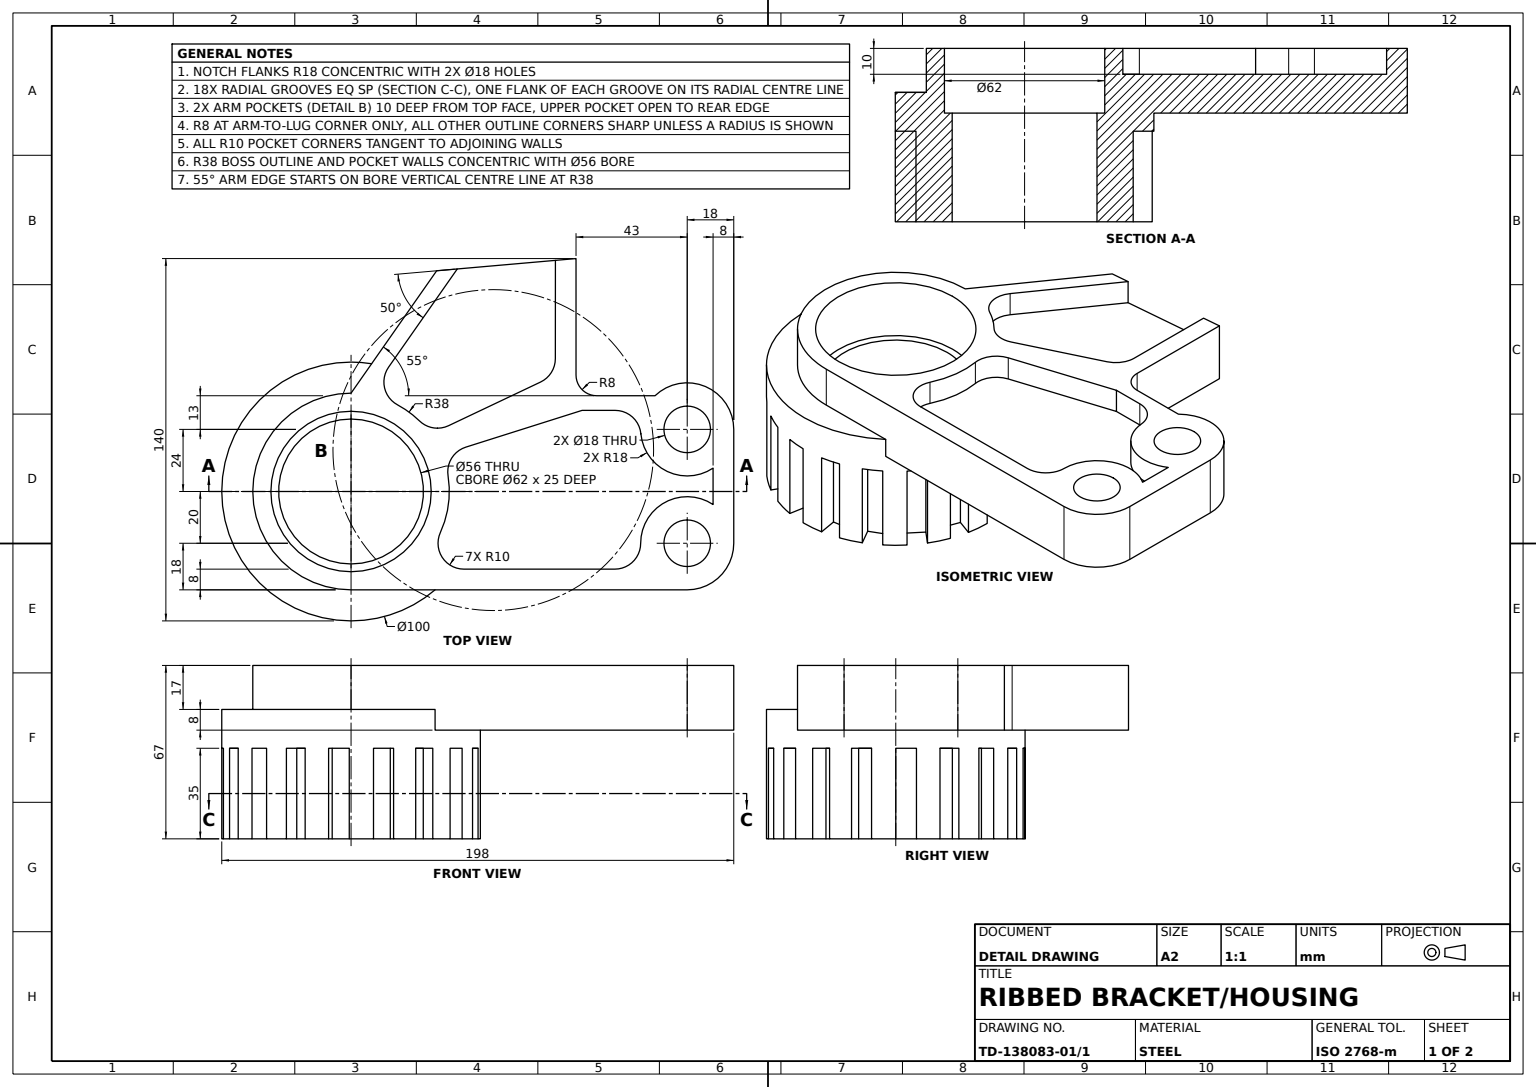
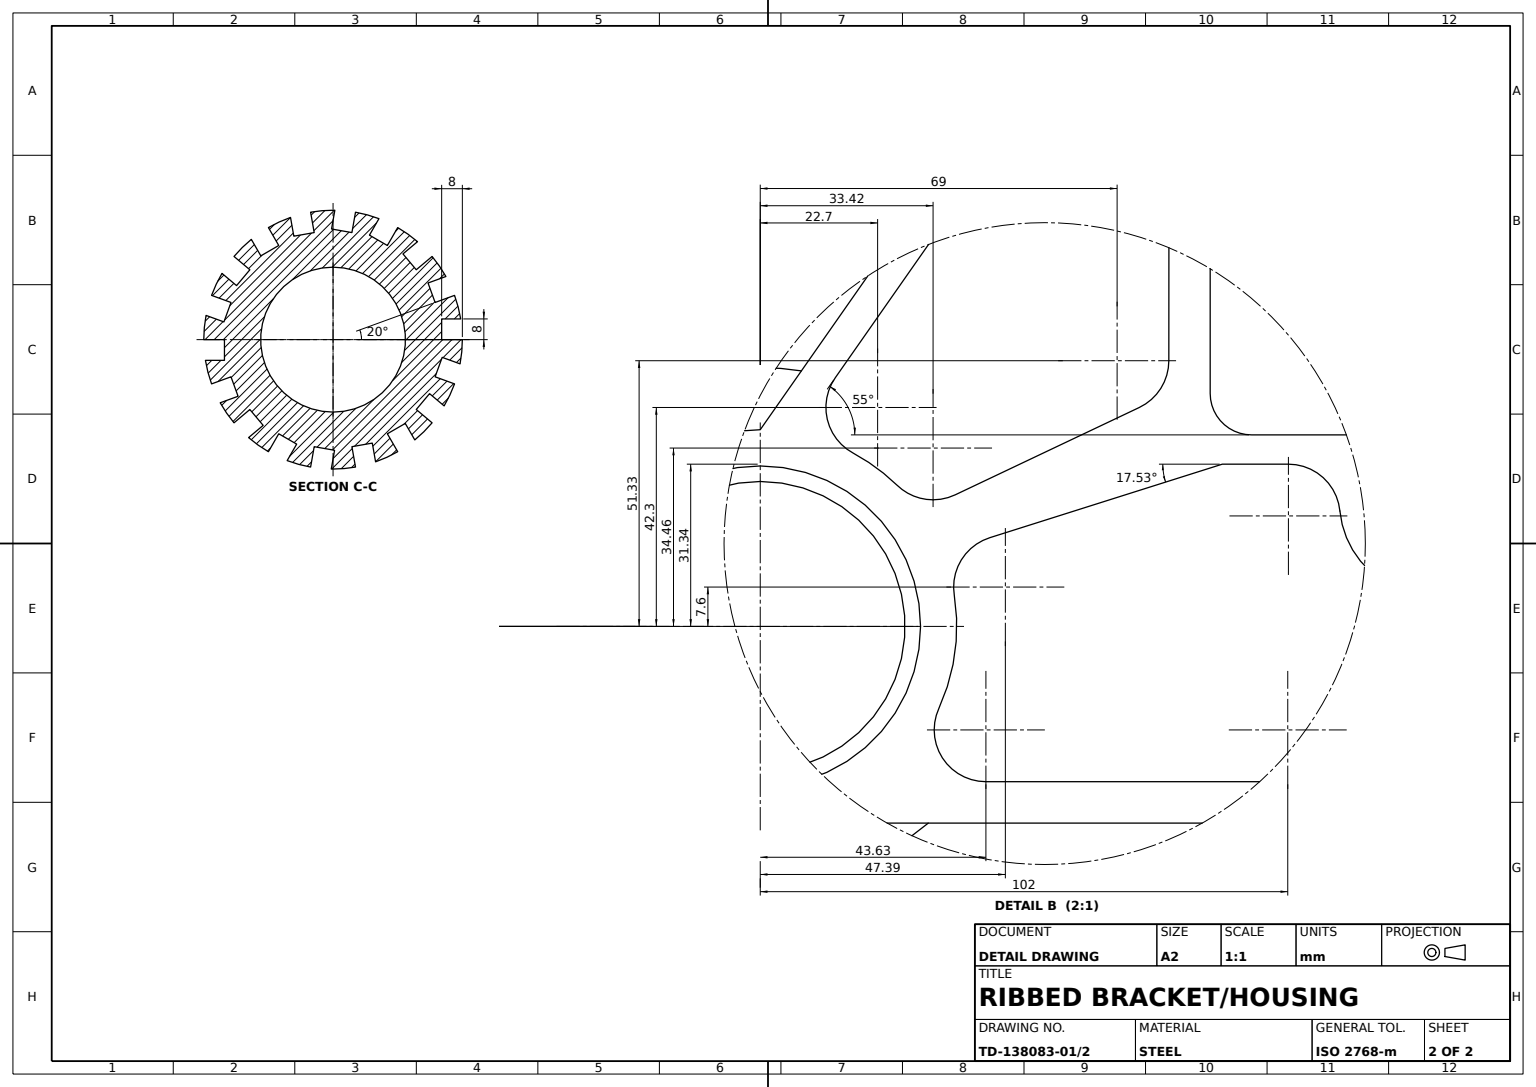
solid
v1 (21,0,-36.373067)
v2 (25,0,-43.30127)
e1 v1 v2 LINE
v3 (21,35,-36.373067)
e2 v3 v1 LINE
v4 (25,35,-43.30127)
e3 v3 v4 LINE
e4 v4 v2 LINE
face PLANE(AX(P(21,0,-36.373067),D(0.866025404,0,0.5),D(0.5,0,-0.866025404))) rev [-e1 -e2 e3 e4]
v5 (102.126336,57,-31.343146)
v6 (102.126336,67,-31.343146)
e5 v5 v6 LINE
v7 (112.081216,57,-22.292022)
e6 v7 v5 CIRCLE(AX(P(102.126336,57,-21.343146),D(0,1,0),D(0,0,1)),10)
v8 (112.081216,67,-22.292022)
e7 v8 v7 LINE
e8 v8 v6 CIRCLE(AX(P(102.126336,67,-21.343146),D(0,1,0),D(0,0,1)),10)
face CYL(AX(P(102.126336,57,-21.343146),D(0,1,0),D(0,0,1)),10) rev [-e5 -e6 -e7 e8]
v9 (21,0,36.373067)
v10 (27.928203,0,32.373067)
e9 v9 v10 LINE
v11 (27.928203,35,32.373067)
e10 v10 v11 LINE
v12 (21,35,36.373067)
e11 v11 v12 LINE
e12 v12 v9 LINE
face PLANE(AX(P(21,0,36.373067),D(-0.5,0,-0.866025404),D(-0.866025404,0,0.5))) rev [e9 e10 e11 e12]
v13 (-14.071797,0,40.373067)
v14 (-14.071797,35,40.373067)
e13 v13 v14 LINE
v15 (-17.749722,0,46.743421)
e14 v13 v15 LINE
v16 (-17.749722,35,46.743421)
e15 v16 v15 LINE
e16 v14 v16 LINE
face PLANE(AX(P(-14.071797,35,40.373067),D(0.866025404,0,0.5),D(0.5,0,-0.866025404))) rev [-e13 e14 -e15 -e16]
v17 (0,42,28)
v18 (0,42,-28)
e17 v17 v18 CIRCLE(AX(P(0,42,0),D(0,1,0),D(0,0,1)),28)
e18 v18 v17 CIRCLE(AX(P(0,42,0),D(0,1,0),D(0,0,1)),28)
v19 (0,42,31)
v20 (0,42,-31)
e19 v19 v20 CIRCLE(AX(P(0,42,0),D(0,1,0),D(0,0,1)),31)
e20 v20 v19 CIRCLE(AX(P(0,42,0),D(0,1,0),D(0,0,1)),31)
face PLANE(AX(P(0,42,0),D(0,1,0),D(0,0,1))) [-e17 -e18] [e19 e20]
v21 (148,42,-24)
v22 (117.5501,42,-37)
e21 v21 v22 CIRCLE(AX(P(130,42,-24),D(0,1,0),D(0,0,1)),18)
v23 (117.5501,67,-37)
e22 v22 v23 LINE
v24 (148,67,-24)
e23 v24 v23 CIRCLE(AX(P(130,67,-24),D(0,1,0),D(0,0,1)),18)
e24 v21 v24 LINE
face CYL(AX(P(130,42,-24),D(0,1,0),D(0,0,1)),18) [e21 e22 -e23 -e24]
v25 (-15.171685,0,-39.97274)
v26 (-15.171685,35,-39.97274)
e25 v25 v26 LINE
v27 (-16.449016,0,-47.216839)
e26 v25 v27 LINE
v28 (-16.449016,35,-47.216839)
e27 v28 v27 LINE
e28 v26 v28 LINE
face PLANE(AX(P(-15.171685,35,-39.97274),D(-0.984807753,0,0.173648178),D(0.173648178,0,0.984807753))) rev [-e25 e26 -e27 -e28]
v29 (-27.928203,35,-32.373067)
v30 (-21,35,-36.373067)
e29 v29 v30 LINE
v31 (-31.606129,35,-38.743421)
e30 v29 v31 LINE
v32 (-25,35,-43.30127)
e31 v32 v31 CIRCLE(AX(P(0,35,0),D(0,1,0),D(0,0,1)),50)
e32 v30 v32 LINE
face PLANE(AX(P(-21,35,-36.373067),D(0,1,0),D(0,0,1))) rev [-e29 e30 -e31 -e32]
v33 (-46.984631,35,-17.101007)
v34 (-49.11549,35,-9.363154)
e33 v33 v34 CIRCLE(AX(P(0,35,0),D(0,1,0),D(0,0,1)),50)
v35 (-39.46709,35,-14.364846)
e34 v35 v33 LINE
v36 (-42.203251,35,-6.847305)
e35 v36 v35 LINE
e36 v36 v34 LINE
face PLANE(AX(P(-39.46709,35,-14.364846),D(0,1,0),D(0,0,1))) rev [-e33 -e34 -e35 e36]
v37 (-21,0,36.373067)
e37 v37 v13 LINE
v38 (-21,35,36.373067)
e38 v14 v38 LINE
e39 v38 v37 LINE
face PLANE(AX(P(-21,0,36.373067),D(0.5,0,-0.866025404),D(-0.866025404,0,-0.5))) rev [e37 e13 e38 e39]
v39 (0.585239,0,42.751111)
v40 (0.585239,35,42.751111)
e40 v39 v40 LINE
v41 (-0.692092,0,49.99521)
e41 v39 v41 LINE
v42 (-0.692092,35,49.99521)
e42 v42 v41 LINE
e43 v40 v42 LINE
face PLANE(AX(P(0.585239,35,42.751111),D(0.984807753,0,0.173648178),D(0.173648178,0,-0.984807753))) rev [-e40 e41 -e42 -e43]
v43 (87,42,-90)
v44 (87,67,-90)
e44 v43 v44 LINE
v45 (33.109445,42,-85.285187)
e45 v43 v45 LINE
v46 (33.109445,67,-85.285187)
e46 v45 v46 LINE
v47 (41.079002,67,-85.982433)
e47 v47 v46 LINE
v48 (41.079002,57,-85.982433)
e48 v48 v47 LINE
v49 (79.030442,57,-89.302754)
e49 v49 v48 LINE
v50 (79.030442,67,-89.302754)
e50 v49 v50 LINE
e51 v44 v50 LINE
face PLANE(AX(P(-7.153305,42,-81.762653),D(-0.087155743,0,-0.996194698),D(-0.996194698,0,0.087155743))) [-e44 e45 e46 -e47 -e48 -e49 e50 -e51]
v51 (140,57,5.03337)
v52 (112,57,20)
e52 v51 v52 CIRCLE(AX(P(130,57,20),D(0,1,0),D(0,0,1)),18)
v53 (112,67,20)
e53 v52 v53 LINE
v54 (140,67,5.03337)
e54 v54 v53 CIRCLE(AX(P(130,67,20),D(0,1,0),D(0,0,1)),18)
e55 v51 v54 LINE
face CYL(AX(P(130,57,20),D(0,1,0),D(0,0,1)),18) [e52 e53 -e54 -e55]
v55 (32.173867,0,-26.99708)
v56 (27.031566,0,-33.125435)
e56 v55 v56 LINE
v57 (27.031566,35,-33.125435)
e57 v56 v57 LINE
v58 (32.173867,35,-26.99708)
e58 v57 v58 LINE
e59 v58 v55 LINE
face PLANE(AX(P(32.173867,0,-26.99708),D(-0.766044443,0,0.64278761),D(0.64278761,0,0.766044443))) rev [e56 e57 e58 e59]
v59 (102,57,30)
e60 v59 v52 CIRCLE(AX(P(102,57,20),D(0,1,0),D(0,0,1)),10)
v60 (102,67,30)
e61 v60 v59 LINE
e62 v60 v53 CIRCLE(AX(P(102,67,20),D(0,1,0),D(0,0,1)),10)
face CYL(AX(P(102,57,20),D(0,1,0),D(0,0,1)),10) rev [-e60 -e61 e62 -e53]
v61 (7.293223,0,41.361926)
v62 (8.682409,0,49.240388)
e63 v61 v62 LINE
v63 (0,0,50)
e64 v63 v62 CIRCLE(AX(P(0,0,0),D(0,1,0),D(0,0,1)),50)
e65 v41 v63 CIRCLE(AX(P(0,0,0),D(0,1,0),D(0,0,1)),50)
v64 (-7.293223,0,41.361926)
e66 v64 v39 LINE
v65 (-8.682409,0,49.240388)
e67 v64 v65 LINE
e68 v15 v65 CIRCLE(AX(P(0,0,0),D(0,1,0),D(0,0,1)),50)
v66 (-25,0,43.30127)
e69 v37 v66 LINE
v67 (-32.666474,0,37.853685)
e70 v67 v66 CIRCLE(AX(P(0,0,0),D(0,1,0),D(0,0,1)),50)
v68 (-27.031566,0,33.125435)
e71 v68 v67 LINE
v69 (-32.173867,0,26.99708)
e72 v69 v68 LINE
v70 (-38.302222,0,32.13938)
e73 v69 v70 LINE
v71 (-43.643168,0,24.398236)
e74 v71 v70 CIRCLE(AX(P(0,0,0),D(0,1,0),D(0,0,1)),50)
v72 (-36.730929,0,21.882387)
e75 v72 v71 LINE
v73 (-39.46709,0,14.364846)
e76 v73 v72 LINE
v74 (-46.984631,0,17.101007)
e77 v73 v74 LINE
v75 (-49.355851,0,8)
e78 v75 v74 CIRCLE(AX(P(0,0,0),D(0,1,0),D(0,0,1)),50)
v76 (-42,0,8)
e79 v76 v75 LINE
v77 (-42,0,0)
e80 v77 v76 LINE
v78 (-50,0,0)
e81 v77 v78 LINE
v79 (-49.11549,0,-9.363154)
e82 v79 v78 CIRCLE(AX(P(0,0,0),D(0,1,0),D(0,0,1)),50)
v80 (-42.203251,0,-6.847305)
e83 v80 v79 LINE
v81 (-39.46709,0,-14.364846)
e84 v81 v80 LINE
v82 (-46.984631,0,-17.101007)
e85 v81 v82 LINE
v83 (-42.951076,0,-25.596974)
e86 v83 v82 CIRCLE(AX(P(0,0,0),D(0,1,0),D(0,0,1)),50)
v84 (-37.316167,0,-20.868724)
e87 v84 v83 LINE
v85 (-32.173867,0,-26.99708)
e88 v85 v84 LINE
v86 (-38.302222,0,-32.13938)
e89 v85 v86 LINE
v87 (-31.606129,0,-38.743421)
e90 v87 v86 CIRCLE(AX(P(0,0,0),D(0,1,0),D(0,0,1)),50)
v88 (-27.928203,0,-32.373067)
e91 v88 v87 LINE
v89 (-21,0,-36.373067)
e92 v89 v88 LINE
v90 (-25,0,-43.30127)
e93 v89 v90 LINE
e94 v27 v90 CIRCLE(AX(P(0,0,0),D(0,1,0),D(0,0,1)),50)
v91 (-7.293223,0,-41.361926)
e95 v91 v25 LINE
v92 (-8.682409,0,-49.240388)
e96 v91 v92 LINE
v93 (0,0,-50)
e97 v93 v92 CIRCLE(AX(P(0,0,0),D(0,1,0),D(0,0,1)),50)
v94 (0.692092,0,-49.99521)
e98 v94 v93 CIRCLE(AX(P(0,0,0),D(0,1,0),D(0,0,1)),50)
v95 (-0.585239,0,-42.751111)
e99 v95 v94 LINE
v96 (7.293223,0,-41.361926)
e100 v96 v95 LINE
v97 (8.682409,0,-49.240388)
e101 v96 v97 LINE
v98 (17.749722,0,-46.743421)
e102 v98 v97 CIRCLE(AX(P(0,0,0),D(0,1,0),D(0,0,1)),50)
v99 (14.071797,0,-40.373067)
e103 v99 v98 LINE
e104 v1 v99 LINE
v100 (32.666474,0,-37.853685)
e105 v100 v2 CIRCLE(AX(P(0,0,0),D(0,1,0),D(0,0,1)),50)
e106 v56 v100 LINE
v101 (38.302222,0,-32.13938)
e107 v55 v101 LINE
v102 (43.643168,0,-24.398236)
e108 v102 v101 CIRCLE(AX(P(0,0,0),D(0,1,0),D(0,0,1)),50)
v103 (36.730929,0,-21.882387)
e109 v103 v102 LINE
v104 (39.46709,0,-14.364846)
e110 v104 v103 LINE
v105 (46.984631,0,-17.101007)
e111 v104 v105 LINE
v106 (49.355851,0,-8)
e112 v106 v105 CIRCLE(AX(P(0,0,0),D(0,1,0),D(0,0,1)),50)
v107 (42,0,-8)
e113 v107 v106 LINE
v108 (42,0,0)
e114 v108 v107 LINE
v109 (50,0,0)
e115 v108 v109 LINE
v110 (49.11549,0,9.363154)
e116 v110 v109 CIRCLE(AX(P(0,0,0),D(0,1,0),D(0,0,1)),50)
v111 (42.203251,0,6.847305)
e117 v111 v110 LINE
v112 (39.46709,0,14.364846)
e118 v112 v111 LINE
v113 (46.984631,0,17.101007)
e119 v112 v113 LINE
v114 (42.951076,0,25.596974)
e120 v114 v113 CIRCLE(AX(P(0,0,0),D(0,1,0),D(0,0,1)),50)
v115 (37.316167,0,20.868724)
e121 v115 v114 LINE
v116 (32.173867,0,26.99708)
e122 v116 v115 LINE
v117 (38.302222,0,32.13938)
e123 v116 v117 LINE
v118 (31.606129,0,38.743421)
e124 v118 v117 CIRCLE(AX(P(0,0,0),D(0,1,0),D(0,0,1)),50)
e125 v10 v118 LINE
v119 (25,0,43.30127)
e126 v9 v119 LINE
v120 (16.449016,0,47.216839)
e127 v120 v119 CIRCLE(AX(P(0,0,0),D(0,1,0),D(0,0,1)),50)
v121 (15.171685,0,39.97274)
e128 v121 v120 LINE
e129 v61 v121 LINE
v122 (0,0,28)
v123 (0,0,-28)
e130 v122 v123 CIRCLE(AX(P(0,0,0),D(0,1,0),D(0,0,1)),28)
e131 v123 v122 CIRCLE(AX(P(0,0,0),D(0,1,0),D(0,0,1)),28)
face PLANE(AX(P(0,0,0),D(0,1,0),D(0,0,1))) rev [e63 -e64 -e65 -e41 -e66 e67 -e68 -e14 -e37 e69 -e70 -e71 -e72 e73 -e74 -e75 -e76 e77 -e78 -e79 -e80 e81 -e82 -e83 -e84 e85 -e86 -e87 -e88 e89 -e90 -e91 -e92 e93 -e94 -e26 -e95 e96 -e97 -e98 -e99 -e100 e101 -e102 -e103 -e104 e1 -e105 -e106 -e56 e107 -e108 -e109 -e110 e111 -e112 -e113 -e114 e115 -e116 -e117 -e118 e119 -e120 -e121 -e122 e123 -e124 -e125 -e9 e126 -e127 -e128 -e129] [e130 e131]
v124 (-37.316167,35,-20.868724)
e132 v84 v124 LINE
v125 (-32.173867,35,-26.99708)
e133 v124 v125 LINE
e134 v125 v85 LINE
face PLANE(AX(P(-32.173867,0,-26.99708),D(0.766044443,0,0.64278761),D(0.64278761,0,-0.766044443))) rev [e88 e132 e133 e134]
v126 (0,67,-31)
e135 v20 v126 LINE
v127 (0,67,31)
e136 v126 v127 CIRCLE(AX(P(0,67,0),D(0,1,0),D(0,0,1)),31)
e137 v19 v127 LINE
face CYL(AX(P(0,42,0),D(0,1,0),D(0,0,1)),31) rev [-e20 e135 e136 -e137]
v128 (-38.302222,35,32.13938)
v129 (-32.666474,35,37.853685)
e138 v128 v129 CIRCLE(AX(P(0,35,0),D(0,1,0),D(0,0,1)),50)
e139 v129 v67 LINE
v130 (-25,35,43.30127)
e140 v130 v66 LINE
e141 v130 v16 CIRCLE(AX(P(0,35,0),D(0,1,0),D(0,0,1)),50)
v131 (-8.682409,35,49.240388)
e142 v131 v65 LINE
e143 v131 v42 CIRCLE(AX(P(0,35,0),D(0,1,0),D(0,0,1)),50)
v132 (0,50,50)
e144 v132 v63 LINE
v133 (0,50,-50)
e145 v133 v132 CIRCLE(AX(P(0,50,0),D(0,1,0),D(0,0,1)),50)
e146 v133 v93 LINE
v134 (-8.682409,35,-49.240388)
e147 v134 v92 LINE
e148 v134 v28 CIRCLE(AX(P(0,35,0),D(0,1,0),D(0,0,1)),50)
e149 v32 v90 LINE
e150 v31 v87 LINE
v135 (-38.302222,35,-32.13938)
e151 v135 v86 LINE
v136 (-42.951076,35,-25.596974)
e152 v135 v136 CIRCLE(AX(P(0,35,0),D(0,1,0),D(0,0,1)),50)
e153 v136 v83 LINE
e154 v33 v82 LINE
e155 v34 v79 LINE
v137 (-50,35,0)
e156 v137 v78 LINE
v138 (-49.355851,35,8)
e157 v137 v138 CIRCLE(AX(P(0,35,0),D(0,1,0),D(0,0,1)),50)
e158 v138 v75 LINE
v139 (-46.984631,35,17.101007)
e159 v139 v74 LINE
v140 (-43.643168,35,24.398236)
e160 v139 v140 CIRCLE(AX(P(0,35,0),D(0,1,0),D(0,0,1)),50)
e161 v140 v71 LINE
e162 v128 v70 LINE
face CYL(AX(P(0,50,0),D(0,-1,0),D(0,0,-1)),50) [e138 e139 e70 -e140 e141 e15 e68 -e142 e143 e42 e65 -e144 -e145 e146 e97 -e147 e148 e27 e94 -e149 e31 e150 e90 -e151 e152 e153 e86 -e154 e33 e155 e82 -e156 e157 e158 e78 -e159 e160 e161 e74 -e162]
e163 v127 v126 CIRCLE(AX(P(0,67,0),D(0,1,0),D(0,0,1)),31)
face CYL(AX(P(0,42,0),D(0,1,0),D(0,0,1)),31) rev [e163 -e135 -e19 e137]
e164 v125 v135 LINE
e165 v124 v136 LINE
face PLANE(AX(P(-32.173867,35,-26.99708),D(0,1,0),D(0,0,1))) rev [-e152 -e164 -e133 e165]
v141 (14.071797,35,-40.373067)
e166 v141 v3 LINE
e167 v99 v141 LINE
face PLANE(AX(P(21,0,-36.373067),D(-0.5,0,0.866025404),D(0.866025404,0,0.5))) rev [e166 e2 e104 e167]
v142 (42,35,-8)
v143 (42,35,0)
e168 v142 v143 LINE
e169 v143 v108 LINE
e170 v107 v142 LINE
face PLANE(AX(P(42,0,0),D(-1,0,0),D(0,0,1))) rev [e168 e169 e114 e170]
v144 (95,42,-37)
e171 v22 v144 LINE
v145 (95,67,-37)
e172 v144 v145 LINE
e173 v23 v145 LINE
face PLANE(AX(P(0,42,-37),D(0,0,-1),D(-1,0,0))) [-e22 e171 e172 -e173]
v146 (-7.293223,35,41.361926)
e174 v146 v64 LINE
e175 v40 v146 LINE
face PLANE(AX(P(-7.293223,0,41.361926),D(0.173648178,0,-0.984807753),D(-0.984807753,0,-0.173648178))) rev [e174 e66 e40 e175]
v147 (38.302222,35,32.13938)
v148 (42.951076,35,25.596974)
e176 v147 v148 CIRCLE(AX(P(0,35,0),D(0,1,0),D(0,0,1)),50)
v149 (32.173867,35,26.99708)
e177 v149 v147 LINE
v150 (37.316167,35,20.868724)
e178 v150 v149 LINE
e179 v150 v148 LINE
face PLANE(AX(P(32.173867,35,26.99708),D(0,1,0),D(0,0,1))) rev [-e176 -e177 -e178 e179]
v151 (46.984631,35,17.101007)
v152 (49.11549,35,9.363154)
e180 v151 v152 CIRCLE(AX(P(0,35,0),D(0,1,0),D(0,0,1)),50)
v153 (39.46709,35,14.364846)
e181 v153 v151 LINE
v154 (42.203251,35,6.847305)
e182 v154 v153 LINE
e183 v154 v152 LINE
face PLANE(AX(P(39.46709,35,14.364846),D(0,1,0),D(0,0,1))) rev [-e180 -e181 -e182 e183]
v155 (130,57,-6)
v156 (130,67,-6)
e184 v155 v156 LINE
v157 (140,57,-9.03337)
e185 v155 v157 CIRCLE(AX(P(130,57,-24),D(0,1,0),D(0,0,1)),18)
v158 (140,67,-9.03337)
e186 v157 v158 LINE
e187 v156 v158 CIRCLE(AX(P(130,67,-24),D(0,1,0),D(0,0,1)),18)
face CYL(AX(P(130,57,-24),D(0,1,0),D(0,0,1)),18) [-e184 e185 e186 -e187]
v159 (-7.293223,35,-41.361926)
e188 v159 v91 LINE
e189 v159 v134 LINE
face PLANE(AX(P(-7.293223,0,-41.361926),D(0.984807753,0,-0.173648178),D(-0.173648178,0,-0.984807753))) rev [-e188 e189 e147 -e96]
v160 (148,67,20)
e190 v160 v24 LINE
v161 (148,42,20)
e191 v161 v160 LINE
e192 v161 v21 LINE
face PLANE(AX(P(148,42,0),D(1,0,0),D(0,0,-1))) [-e190 -e191 e192 e24]
v162 (32.666474,35,-37.853685)
e193 v162 v100 LINE
e194 v57 v162 LINE
face PLANE(AX(P(27.031566,35,-33.125435),D(-0.64278761,0,-0.766044443),D(-0.766044443,0,0.64278761))) rev [-e193 -e194 -e57 e106]
v163 (-42,35,8)
v164 (-42,35,0)
e195 v163 v164 LINE
e196 v163 v138 LINE
e197 v164 v137 LINE
face PLANE(AX(P(-42,35,0),D(0,1,0),D(0,0,1))) rev [-e195 e196 -e157 -e197]
e198 v164 v77 LINE
face PLANE(AX(P(-42,0,0),D(0,0,-1),D(-1,0,0))) rev [e156 -e81 -e198 e197]
v165 (8.682409,35,-49.240388)
e199 v165 v97 LINE
v166 (7.293223,35,-41.361926)
e200 v166 v96 LINE
e201 v166 v165 LINE
face PLANE(AX(P(7.293223,0,-41.361926),D(0.984807753,0,0.173648178),D(0.173648178,0,-0.984807753))) rev [e199 -e101 -e200 e201]
v167 (89.343146,57,-31.343146)
v168 (44.381437,57,-17.136695)
e202 v167 v168 LINE
v169 (89.343146,67,-31.343146)
e203 v167 v169 LINE
v170 (44.381437,67,-17.136695)
e204 v169 v170 LINE
e205 v170 v168 LINE
face PLANE(AX(P(-0.894492,57,-2.830961),D(-0.301285958,0,-0.953533834),D(-0.953533834,0,0.301285958))) rev [-e202 e203 e204 e205]
v171 (37.520485,57,-6.017741)
e206 v168 v171 CIRCLE(AX(P(47.394297,57,-7.601357),D(0,1,0),D(0,0,1)),10)
v172 (34.544255,57,15.833333)
e207 v172 v171 CIRCLE(AX(P(0,57,0),D(0,1,0),D(0,0,1)),38)
v173 (43.634848,57,30)
e208 v172 v173 CIRCLE(AX(P(43.634848,57,20),D(0,1,0),D(0,0,1)),10)
e209 v59 v173 LINE
e210 v157 v51 LINE
e211 v7 v155 CIRCLE(AX(P(130,57,-24),D(0,1,0),D(0,0,1)),18)
e212 v167 v5 LINE
face PLANE(AX(P(0,57,0),D(0,1,0),D(0,0,1))) [e202 e206 -e207 e208 -e209 e60 -e52 -e210 -e185 -e211 e6 -e212]
e213 v153 v112 LINE
e214 v151 v113 LINE
face PLANE(AX(P(39.46709,0,14.364846),D(-0.342020143,0,0.939692621),D(0.939692621,0,0.342020143))) rev [-e119 -e213 e181 e214]
v174 (39.46709,35,-14.364846)
v175 (46.984631,35,-17.101007)
e215 v174 v175 LINE
e216 v175 v105 LINE
e217 v174 v104 LINE
face PLANE(AX(P(39.46709,0,-14.364846),D(0.342020143,0,0.939692621),D(0.939692621,0,-0.342020143))) rev [e215 e216 -e111 -e217]
v176 (130,67,-15)
v177 (130,67,-33)
e218 v176 v177 CIRCLE(AX(P(130,67,-24),D(0,1,0),D(0,0,1)),9)
v178 (130,42,-33)
e219 v178 v177 LINE
v179 (130,42,-15)
e220 v179 v178 CIRCLE(AX(P(130,42,-24),D(0,1,0),D(0,0,1)),9)
e221 v179 v176 LINE
face CYL(AX(P(130,42,-24),D(0,1,0),D(0,0,1)),9) rev [e218 -e219 -e220 e221]
v180 (-0.585239,35,-42.751111)
e222 v95 v180 LINE
e223 v180 v166 LINE
face PLANE(AX(P(7.293223,0,-41.361926),D(-0.173648178,0,0.984807753),D(0.984807753,0,0.173648178))) rev [e222 e223 e200 e100]
v181 (130,42,29)
v182 (130,67,29)
e224 v181 v182 LINE
v183 (130,42,11)
e225 v183 v181 CIRCLE(AX(P(130,42,20),D(0,1,0),D(0,0,1)),9)
v184 (130,67,11)
e226 v183 v184 LINE
e227 v184 v182 CIRCLE(AX(P(130,67,20),D(0,1,0),D(0,0,1)),9)
face CYL(AX(P(130,42,20),D(0,1,0),D(0,0,1)),9) rev [-e224 -e225 e226 e227]
e228 v76 v163 LINE
face PLANE(AX(P(-42,35,8),D(0,0,1),D(1,0,0))) rev [-e158 -e196 -e228 e79]
v185 (50,35,0)
e229 v143 v185 LINE
e230 v185 v109 LINE
face PLANE(AX(P(42,0,0),D(0,0,1),D(1,0,0))) rev [-e169 e229 e230 -e115]
e231 v181 v183 CIRCLE(AX(P(130,42,20),D(0,1,0),D(0,0,1)),9)
v186 (87,42,-45)
e232 v186 v43 LINE
e233 v144 v186 CIRCLE(AX(P(95,42,-45),D(0,-1,0),D(0,0,1)),8)
v187 (130,42,38)
e234 v187 v161 CIRCLE(AX(P(130,42,20),D(0,1,0),D(0,0,1)),18)
v188 (32.496154,42,38)
e235 v188 v187 LINE
v189 (7.956388,42,-49.3629)
e236 v188 v189 CIRCLE(AX(P(0,42,0),D(0,1,0),D(0,0,1)),50)
e237 v189 v45 LINE
e238 v178 v179 CIRCLE(AX(P(130,42,-24),D(0,1,0),D(0,0,1)),9)
face PLANE(AX(P(0,42,0),D(0,1,0),D(0,0,1))) rev [e231 e225] [-e232 -e233 -e171 -e21 -e192 -e234 -e235 e236 e237 -e45] [e220 e238]
e239 v182 v184 CIRCLE(AX(P(130,67,20),D(0,1,0),D(0,0,1)),9)
face CYL(AX(P(130,42,20),D(0,1,0),D(0,0,1)),9) rev [e239 -e226 -e231 e224]
v190 (32.496154,50,38)
e240 v188 v190 LINE
e241 v132 v190 CIRCLE(AX(P(0,50,0),D(0,1,0),D(0,0,1)),50)
v191 (8.682409,35,49.240388)
e242 v191 v62 LINE
v192 (16.449016,35,47.216839)
e243 v191 v192 CIRCLE(AX(P(0,35,0),D(0,1,0),D(0,0,1)),50)
e244 v192 v120 LINE
v193 (25,35,43.30127)
e245 v193 v119 LINE
v194 (31.606129,35,38.743421)
e246 v193 v194 CIRCLE(AX(P(0,35,0),D(0,1,0),D(0,0,1)),50)
e247 v194 v118 LINE
e248 v147 v117 LINE
e249 v148 v114 LINE
e250 v152 v110 LINE
v195 (49.355851,35,-8)
e251 v185 v195 CIRCLE(AX(P(0,35,0),D(0,1,0),D(0,0,1)),50)
e252 v195 v106 LINE
v196 (43.643168,35,-24.398236)
e253 v175 v196 CIRCLE(AX(P(0,35,0),D(0,1,0),D(0,0,1)),50)
e254 v196 v102 LINE
v197 (38.302222,35,-32.13938)
e255 v197 v101 LINE
e256 v197 v162 CIRCLE(AX(P(0,35,0),D(0,1,0),D(0,0,1)),50)
v198 (17.749722,35,-46.743421)
e257 v4 v198 CIRCLE(AX(P(0,35,0),D(0,1,0),D(0,0,1)),50)
e258 v198 v98 LINE
v199 (0.692092,35,-49.99521)
e259 v165 v199 CIRCLE(AX(P(0,35,0),D(0,1,0),D(0,0,1)),50)
e260 v199 v94 LINE
v200 (7.956388,50,-49.3629)
e261 v200 v133 CIRCLE(AX(P(0,50,0),D(0,1,0),D(0,0,1)),50)
e262 v189 v200 LINE
face CYL(AX(P(0,50,0),D(0,-1,0),D(0,0,-1)),50) [e240 -e241 e144 e64 -e242 e243 e244 e127 -e245 e246 e247 e124 -e248 e176 e249 e120 -e214 e180 e250 e116 -e230 e251 e252 e112 -e216 e253 e254 e108 -e255 e256 e193 e105 -e4 e257 e258 e102 -e199 e259 e260 e98 -e146 -e261 -e262 -e236]
e263 v11 v194 LINE
e264 v12 v193 LINE
face PLANE(AX(P(21,35,36.373067),D(0,1,0),D(0,0,1))) rev [-e11 e263 -e246 -e264]
v201 (36.730929,35,-21.882387)
e265 v201 v196 LINE
e266 v201 v174 LINE
face PLANE(AX(P(39.46709,35,-14.364846),D(0,1,0),D(0,0,1))) rev [e265 -e253 -e215 -e266]
v202 (15.171685,35,39.97274)
e267 v202 v192 LINE
e268 v121 v202 LINE
face PLANE(AX(P(15.171685,35,39.97274),D(0.984807753,0,-0.173648178),D(-0.173648178,0,-0.984807753))) rev [e128 -e244 -e267 -e268]
v203 (43.634848,67,30)
e269 v173 v203 LINE
e270 v60 v203 LINE
face PLANE(AX(P(0,57,30),D(0,0,-1),D(-1,0,0))) [e209 e269 -e270 e61]
v204 (26.456469,57,-27.277376)
v205 (33.418697,57,-24.455633)
e271 v204 v205 CIRCLE(AX(P(33.418697,57,-34.455633),D(0,1,0),D(0,0,1)),10)
v206 (26.456469,67,-27.277376)
e272 v206 v204 LINE
v207 (33.418697,67,-24.455633)
e273 v206 v207 CIRCLE(AX(P(33.418697,67,-34.455633),D(0,1,0),D(0,0,1)),10)
e274 v205 v207 LINE
face CYL(AX(P(33.418697,57,-34.455633),D(0,1,0),D(0,0,1)),10) rev [-e271 -e272 e273 -e274]
v208 (79.004343,57,-51.320958)
v209 (79.004343,67,-51.320958)
e275 v208 v209 LINE
e276 v209 v50 LINE
e277 v208 v49 LINE
face PLANE(AX(P(78.969041,57,0.054263),D(0.999999764,0,0.000687145),D(0.000687145,0,-0.999999764))) rev [e275 e276 -e50 -e277]
v210 (-32.173867,35,26.99708)
e278 v210 v128 LINE
e279 v210 v69 LINE
face PLANE(AX(P(-32.173867,0,26.99708),D(-0.64278761,0,-0.766044443),D(-0.766044443,0,0.64278761))) rev [e278 e162 -e73 -e279]
e280 v142 v195 LINE
face PLANE(AX(P(42,35,0),D(0,1,0),D(0,0,1))) rev [-e168 e280 -e251 -e229]
face PLANE(AX(P(-42,0,0),D(1,0,0),D(0,0,-1))) rev [e228 e195 e198 e80]
e281 v180 v199 LINE
face PLANE(AX(P(-0.585239,35,-42.751111),D(-0.984807753,0,-0.173648178),D(-0.173648178,0,0.984807753))) rev [-e260 -e281 -e222 e99]
v211 (7.293223,35,41.361926)
e282 v211 v61 LINE
e283 v202 v211 LINE
face PLANE(AX(P(7.293223,0,41.361926),D(-0.173648178,0,-0.984807753),D(-0.984807753,0,0.173648178))) rev [e282 e129 e268 e283]
v212 (87,67,-45)
e284 v186 v212 LINE
e285 v145 v212 CIRCLE(AX(P(95,67,-45),D(0,-1,0),D(0,0,1)),8)
face CYL(AX(P(95,42,-45),D(0,1,0),D(0,0,1)),8) rev [-e172 e233 e284 -e285]
e286 v88 v29 LINE
face PLANE(AX(P(-27.928203,35,-32.373067),D(-0.866025404,0,0.5),D(0.5,0,0.866025404))) rev [e91 -e150 -e30 -e286]
v213 (-36.730929,35,21.882387)
e287 v72 v213 LINE
e288 v213 v140 LINE
face PLANE(AX(P(-36.730929,35,21.882387),D(0.342020143,0,0.939692621),D(0.939692621,0,-0.342020143))) rev [-e287 e75 -e161 -e288]
v214 (-27.031566,35,33.125435)
e289 v214 v210 LINE
e290 v68 v214 LINE
face PLANE(AX(P(-32.173867,0,26.99708),D(0.766044443,0,-0.64278761),D(-0.64278761,0,-0.766044443))) rev [e289 e279 e72 e290]
v215 (17.968059,57,-33.483561)
v216 (17.968059,67,-33.483561)
e291 v215 v216 LINE
v217 (14.504975,57,-48.030789)
e292 v217 v215 CIRCLE(AX(P(22.696495,57,-42.295025),D(0,1,0),D(0,0,1)),10)
v218 (14.504975,67,-48.030789)
e293 v218 v217 LINE
e294 v218 v216 CIRCLE(AX(P(22.696495,67,-42.295025),D(0,1,0),D(0,0,1)),10)
face CYL(AX(P(22.696495,57,-42.295025),D(0,1,0),D(0,0,1)),10) rev [-e291 -e292 -e293 e294]
face PLANE(AX(P(-37.316167,35,-20.868724),D(-0.64278761,0,0.766044443),D(0.766044443,0,0.64278761))) rev [-e165 -e132 e87 -e153]
e295 v141 v198 LINE
face PLANE(AX(P(14.071797,35,-40.373067),D(-0.866025404,0,-0.5),D(-0.5,0,0.866025404))) rev [-e167 e103 -e258 -e295]
v219 (34.544255,67,15.833333)
v220 (37.520485,67,-6.017741)
e296 v219 v220 CIRCLE(AX(P(0,67,0),D(0,1,0),D(0,0,1)),38)
e297 v219 v172 LINE
e298 v171 v220 LINE
face CYL(AX(P(0,57,0),D(0,1,0),D(0,0,1)),38) [-e296 e297 e207 e298]
e299 v214 v129 LINE
face PLANE(AX(P(-27.031566,35,33.125435),D(0.64278761,0,0.766044443),D(0.766044443,0,-0.64278761))) rev [-e139 -e299 -e290 e71]
e300 v169 v6 LINE
face PLANE(AX(P(0,57,-31.343146),D(0,0,1),D(1,0,0))) [-e300 -e203 e212 e5]
e301 v47 v218 LINE
e302 v48 v217 LINE
face PLANE(AX(P(-12.834105,57,-8.986537),D(-0.819152044,0,-0.573576436),D(-0.573576436,0,0.819152044))) rev [e301 e293 -e302 e48]
e303 v26 v159 LINE
face PLANE(AX(P(-7.293223,35,-41.361926),D(0,1,0),D(0,0,1))) rev [-e189 -e303 e28 -e148]
face PLANE(AX(P(-7.293223,0,-41.361926),D(0.173648178,0,0.984807753),D(0.984807753,0,-0.173648178))) rev [e25 e303 e188 e95]
face PLANE(AX(P(21,35,-36.373067),D(0,1,0),D(0,0,1))) rev [-e166 e295 -e257 -e3]
e304 v158 v54 LINE
face PLANE(AX(P(140,57,0),D(-1,0,0),D(0,0,1))) [e210 e55 -e304 -e186]
v221 (-39.46709,35,14.364846)
e305 v221 v73 LINE
e306 v221 v139 LINE
face PLANE(AX(P(-39.46709,0,14.364846),D(-0.342020143,0,-0.939692621),D(-0.939692621,0,0.342020143))) rev [-e77 -e305 e306 e159]
e307 v212 v44 LINE
face PLANE(AX(P(87,42,0),D(1,0,0),D(0,0,-1))) [-e307 -e284 e232 e44]
e308 v103 v201 LINE
face PLANE(AX(P(36.730929,35,-21.882387),D(-0.342020143,0,-0.939692621),D(-0.939692621,0,0.342020143))) rev [-e308 e109 -e254 -e265]
e309 v170 v220 CIRCLE(AX(P(47.394297,67,-7.601357),D(0,1,0),D(0,0,1)),10)
face CYL(AX(P(47.394297,57,-7.601357),D(0,1,0),D(0,0,1)),10) rev [-e298 -e206 -e205 e309]
e310 v111 v154 LINE
face PLANE(AX(P(39.46709,0,14.364846),D(-0.939692621,0,-0.342020143),D(-0.342020143,0,0.939692621))) rev [e213 e118 e310 e182]
e311 v146 v131 LINE
face PLANE(AX(P(-7.293223,35,41.361926),D(0,1,0),D(0,0,1))) rev [e43 -e143 -e311 -e175]
e312 v38 v130 LINE
face PLANE(AX(P(-21,0,36.373067),D(-0.866025404,0,-0.5),D(-0.5,0,0.866025404))) rev [-e69 -e39 e312 e140]
e313 v80 v36 LINE
face PLANE(AX(P(-42.203251,35,-6.847305),D(-0.342020143,0,0.939692621),D(0.939692621,0,0.342020143))) rev [-e313 e83 -e155 -e36]
face PLANE(AX(P(42,35,-8),D(0,0,-1),D(-1,0,0))) rev [e113 -e252 -e280 -e170]
e314 v115 v150 LINE
face PLANE(AX(P(37.316167,35,20.868724),D(0.64278761,0,-0.766044443),D(-0.766044443,0,-0.64278761))) rev [-e249 -e179 -e314 e121]
v222 (0,50,38)
v223 (0,67,38)
e315 v222 v223 LINE
e316 v222 v190 LINE
v224 (130,67,38)
e317 v187 v224 LINE
e318 v223 v224 LINE
face PLANE(AX(P(0,42,38),D(0,0,1),D(1,0,0))) [-e315 e316 -e240 e235 e317 -e318]
e319 v122 v17 LINE
e320 v123 v18 LINE
face CYL(AX(P(0,-17,0),D(0,1,0),D(0,0,1)),28) rev [e18 -e319 -e131 e320]
e321 v219 v203 CIRCLE(AX(P(43.634848,67,20),D(0,1,0),D(0,0,1)),10)
face CYL(AX(P(43.634848,57,20),D(0,1,0),D(0,0,1)),10) rev [-e208 -e297 e321 -e269]
face PLANE(AX(P(42.203251,35,6.847305),D(0.342020143,0,-0.939692621),D(-0.939692621,0,-0.342020143))) rev [-e310 e117 -e250 -e183]
e322 v177 v176 CIRCLE(AX(P(130,67,-24),D(0,1,0),D(0,0,1)),9)
face CYL(AX(P(130,42,-24),D(0,1,0),D(0,0,1)),9) rev [e219 e322 -e221 -e238]
e323 v213 v221 LINE
face PLANE(AX(P(-39.46709,35,14.364846),D(0,1,0),D(0,0,1))) rev [-e306 -e323 e288 -e160]
face PLANE(AX(P(-32.173867,35,26.99708),D(0,1,0),D(0,0,1))) rev [-e289 e299 -e138 -e278]
face PLANE(AX(P(27.928203,35,32.373067),D(0.866025404,0,-0.5),D(-0.5,0,-0.866025404))) rev [-e10 e125 -e247 -e263]
v225 (37.702845,57,-25.419811)
v226 (73.288493,57,-42.292008)
e324 v225 v226 LINE
v227 (37.702845,67,-25.419811)
e325 v225 v227 LINE
v228 (73.288493,67,-42.292008)
e326 v227 v228 LINE
e327 v228 v226 LINE
face PLANE(AX(P(-2.920261,57,-6.159209),D(0.428414748,0,0.903582206),D(0.903582206,0,-0.428414748))) rev [-e324 e325 e326 e327]
v229 (0,50,-38)
e328 v229 v200 LINE
e329 v229 v222 CIRCLE(AX(P(0,50,0),D(0,1,0),D(0,0,1)),38)
face PLANE(AX(P(0,50,0),D(0,1,0),D(0,0,1))) [e328 e261 e145 e241 -e316 -e329]
e330 v35 v81 LINE
face PLANE(AX(P(-39.46709,0,-14.364846),D(0.342020143,0,-0.939692621),D(-0.939692621,0,-0.342020143))) rev [e34 e154 -e85 -e330]
face PLANE(AX(P(21,0,36.373067),D(-0.866025404,0,0.5),D(0.5,0,0.866025404))) rev [e264 e245 -e126 -e12]
e331 v211 v191 LINE
face PLANE(AX(P(7.293223,0,41.361926),D(-0.984807753,0,0.173648178),D(0.173648178,0,0.984807753))) rev [e242 -e63 -e282 e331]
face PLANE(AX(P(39.46709,0,-14.364846),D(-0.939692621,0,0.342020143),D(0.342020143,0,0.939692621))) rev [e308 e266 e217 e110]
e332 v30 v89 LINE
face PLANE(AX(P(-21,0,-36.373067),D(0.5,0,0.866025404),D(0.866025404,0,-0.5))) rev [e92 e286 e29 e332]
face PLANE(AX(P(-21,35,36.373067),D(0,1,0),D(0,0,1))) rev [-e312 -e38 e16 -e141]
face CYL(AX(P(0,-17,0),D(0,1,0),D(0,0,1)),28) rev [e319 e17 -e320 -e130]
v230 (0,67,-38)
e333 v230 v223 CIRCLE(AX(P(0,67,0),D(0,1,0),D(0,0,1)),38)
e334 v229 v230 LINE
face CYL(AX(P(0,42,0),D(0,1,0),D(0,0,1)),38) [e315 -e333 -e334 e329]
e335 v206 v216 CIRCLE(AX(P(0,67,0),D(0,1,0),D(0,0,1)),38)
e336 v204 v215 CIRCLE(AX(P(0,57,0),D(0,1,0),D(0,0,1)),38)
face CYL(AX(P(0,57,0),D(0,1,0),D(0,0,1)),38) [-e335 e272 e336 e291]
e337 v8 v156 CIRCLE(AX(P(130,67,-24),D(0,1,0),D(0,0,1)),18)
face CYL(AX(P(130,57,-24),D(0,1,0),D(0,0,1)),18) [-e337 e7 e211 e184]
e338 v205 v225 CIRCLE(AX(P(33.418697,57,-34.455633),D(0,1,0),D(0,0,1)),10)
e339 v226 v208 CIRCLE(AX(P(69.004346,57,-51.32783),D(0,1,0),D(0,0,1)),10)
face PLANE(AX(P(0,57,0),D(0,1,0),D(0,0,1))) [e292 -e336 e271 e338 e324 e339 e277 e49 e302]
e340 v230 v46 LINE
e341 v224 v160 CIRCLE(AX(P(130,67,20),D(0,1,0),D(0,0,1)),18)
e342 v228 v209 CIRCLE(AX(P(69.004346,67,-51.32783),D(0,1,0),D(0,0,1)),10)
e343 v207 v227 CIRCLE(AX(P(33.418697,67,-34.455633),D(0,1,0),D(0,0,1)),10)
face PLANE(AX(P(0,67,0),D(0,1,0),D(0,0,1))) [e335 -e294 -e301 e47 -e340 e333 e318 e341 e190 e23 e173 e285 e307 e51 -e276 -e342 -e326 -e343 -e273] [-e8 e337 e187 e304 e54 -e62 e270 -e321 e296 -e309 -e204 e300] [-e322 -e218] [-e239 -e227] [-e163 -e136]
face PLANE(AX(P(-39.46709,0,-14.364846),D(0.939692621,0,0.342020143),D(0.342020143,0,-0.939692621))) rev [e35 e330 e84 e313]
face PLANE(AX(P(-21,0,-36.373067),D(0.866025404,0,-0.5),D(-0.5,0,-0.866025404))) rev [-e332 e32 e149 -e93]
face PLANE(AX(P(-32.173867,0,-26.99708),D(0.64278761,0,-0.766044443),D(-0.766044443,0,-0.64278761))) rev [-e89 -e134 e164 e151]
face PLANE(AX(P(7.293223,35,-41.361926),D(0,1,0),D(0,0,1))) rev [e281 -e259 -e201 -e223]
face PLANE(AX(P(-17.85416,42,-12.501617),D(0.819152044,0,0.573576436),D(0.573576436,0,-0.819152044))) rev [-e237 e262 -e328 e334 e340 -e46]
face CYL(AX(P(69.004346,57,-51.32783),D(0,1,0),D(0,0,1)),10) rev [e342 -e275 -e339 -e327]
e344 v149 v116 LINE
face PLANE(AX(P(32.173867,0,26.99708),D(-0.64278761,0,0.766044443),D(0.766044443,0,0.64278761))) rev [-e344 e177 e248 -e123]
face PLANE(AX(P(-39.46709,0,14.364846),D(0.939692621,0,-0.342020143),D(-0.342020143,0,-0.939692621))) rev [e76 e287 e323 e305]
face PLANE(AX(P(7.293223,35,41.361926),D(0,1,0),D(0,0,1))) rev [e267 -e243 -e331 -e283]
face CYL(AX(P(130,42,20),D(0,1,0),D(0,0,1)),18) [-e341 -e317 e234 e191]
face PLANE(AX(P(-7.293223,0,41.361926),D(-0.984807753,0,-0.173648178),D(-0.173648178,0,0.984807753))) rev [e311 e142 -e67 -e174]
e345 v58 v197 LINE
face PLANE(AX(P(32.173867,0,-26.99708),D(0.64278761,0,0.766044443),D(0.766044443,0,-0.64278761))) rev [-e107 -e59 e345 e255]
face PLANE(AX(P(32.173867,0,26.99708),D(-0.766044443,0,-0.64278761),D(-0.64278761,0,0.766044443))) rev [e314 e178 e344 e122]
face CYL(AX(P(33.418697,57,-34.455633),D(0,1,0),D(0,0,1)),10) rev [-e338 e274 e343 -e325]
face PLANE(AX(P(32.173867,35,-26.99708),D(0,1,0),D(0,0,1))) rev [e194 -e256 -e345 -e58]
